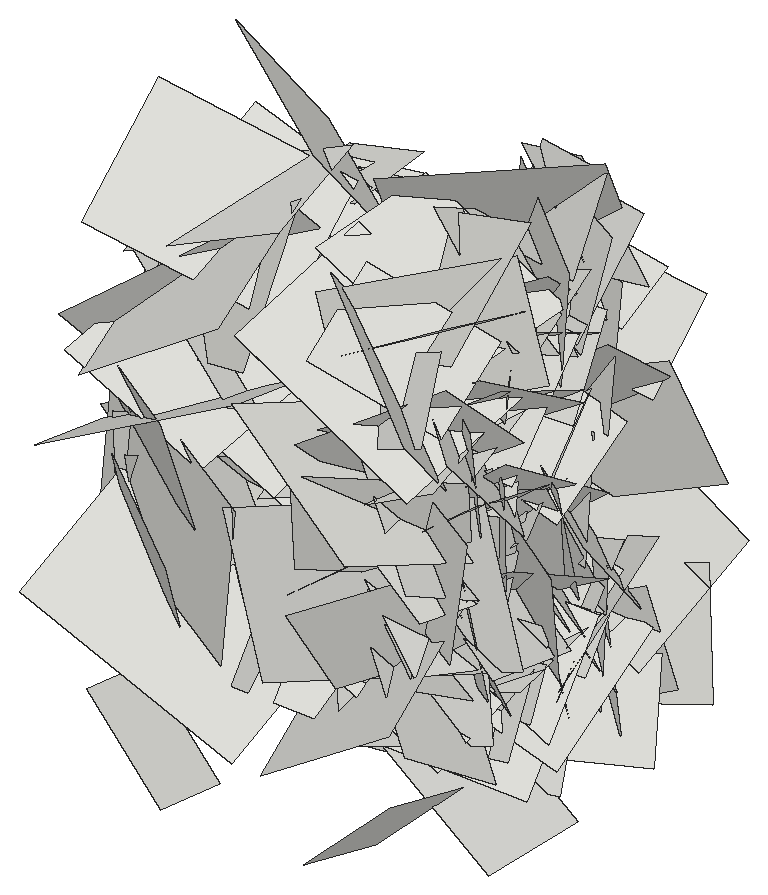
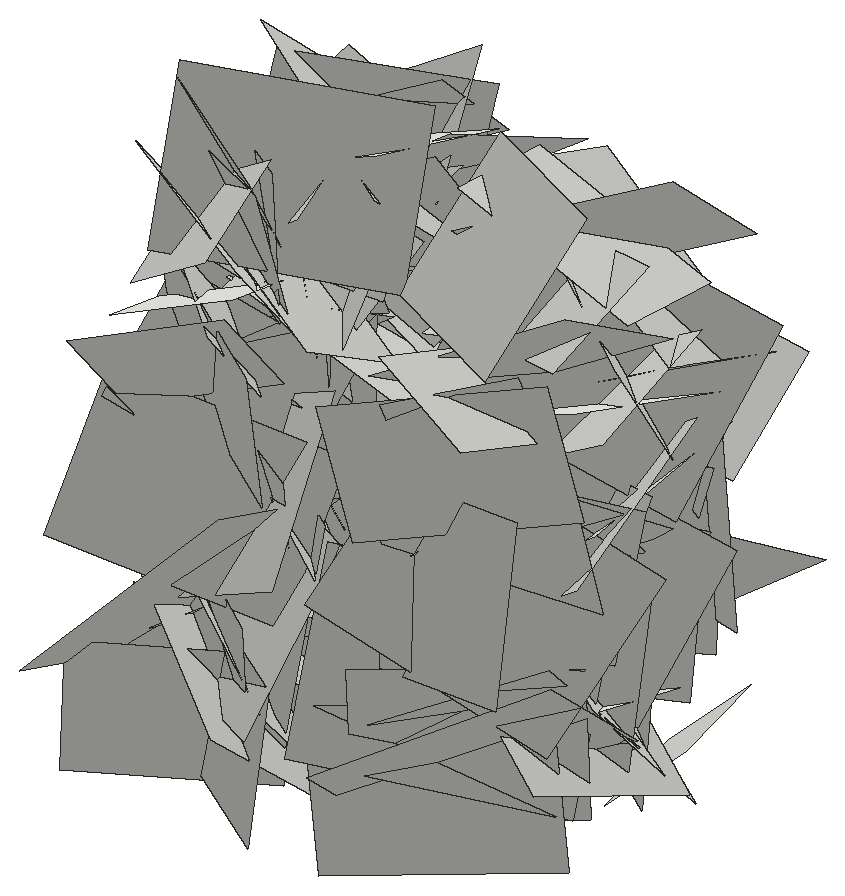
# SketchUp Ruby script. Lengths in inches.
U = 1.inch
M = Sketchup.active_model
def pt(a) = Geom::Point3d.new(a.map { |v| v * U })
def face(e, loops, mat)
  f = e.add_face(loops[0].map { |a| pt(a) })
  loops[1..].each { |l| e.add_face(l.map { |a| pt(a) }).erase! }
  f.material = f.back_material = mat if mat
  f
end
# faces: each face lists its corners as indices into pts; further lists are holes
def faces(e, pts, list, mat = nil) = list.each { |f| face(e, (f[0].is_a?(Array) ? f : [f]).map { |l| l.map { |i| pts[i] } }, mat) }
# xy, xz, yz: faces in a plane at the given z, y or x. An outline is a flat list of corners, or four numbers for a rectangle; further outlines are holes
def ring(l) = l.size == 4 ? [[l[0], l[1]], [l[2], l[1]], [l[2], l[3]], [l[0], l[3]]] : l.each_slice(2).to_a
def flat(e, list, mat, &to3) = list.each { |f| face(e, (f[0].is_a?(Array) ? f : [f]).map { |l| ring(l).map { |u, v| to3.(u, v) } }, mat) }
def xy(e, z, list, mat = nil) = flat(e, list, mat) { |x, y| [x, y, z] }
def xz(e, y, list, mat = nil) = flat(e, list, mat) { |x, z| [x, y, z] }
def yz(e, x, list, mat = nil) = flat(e, list, mat) { |y, z| [x, y, z] }
def lines(e, pts, list) = list.each { |a, b| e.add_line(pt(pts[a]), pt(pts[b])) }
# prism: a flat outline (further loops are holes) pulled along v
def prism(e, loops, v, mat = nil)
  f = face(e, loops, mat); d = Geom::Vector3d.new(v.map { |x| x * U })
  f.pushpull(f.normal.samedirection?(d) ? d.length : -d.length)
end
def box(e, o, s, mat = nil) = prism(e, [[o, [o[0] + s[0], o[1], o[2]], [o[0] + s[0], o[1] + s[1], o[2]], [o[0], o[1] + s[1], o[2]]]], [0, 0, s[2]], mat)
def at(x, y, z, deg = 0) = Geom::Transformation.translation(pt([x, y, z])) * Geom::Transformation.rotation(ORIGIN, Z_AXIS, deg.degrees)
def axes(o, x, y, z) = Geom::Transformation.new([*x, 0, *y, 0, *z, 0, *pt(o).to_a, 1])
def part(name) = M.definitions.add(name)
# library, detail: a bought-in or finely detailed component or shape, given as its bounding box
def library(name, o, s) = part(name).tap { |d| box(d.entities, o, s) }
def detail(e, o, s) = box(e.add_group.entities, o, s)
def put(e, d, t, mat = nil) = e.add_instance(d, t).tap { |i| i.material = mat if mat }
def group(e, t, mat = nil) = e.add_group.tap { |g| g.transformation = t; g.material = mat if mat }.entities
root = M.entities
c1 = part("Component\#6")
p = [[0.01,0,0],[0,3.24,4.54],[4.32,3.24,4.54],[4.33,0,0]]
faces(c1.entities,p,[[0,1,2,3]])
put(root,c1,axes([400.91,193.84,30.46],[0.25587,-1.06575,0.3461],[0.15582,0.3811,1.07099],[1.17751,0.18115,-0.21693]))
put(root,c1,axes([414.68,193.84,30.46],[-0.25587,-1.06575,0.3461],[-0.15582,0.3811,1.07099],[-1.17751,0.18115,-0.21693]))
put(root,c1,axes([404.88,192.39,25.48],[0.15082,-0.34829,0.66058],[0.01541,0.67363,0.35204],[-0.79143,-0.05326,0.13274]))
put(root,c1,axes([410.71,192.39,25.48],[-0.15082,-0.34829,0.66058],[-0.01541,0.67363,0.35204],[0.79143,-0.05326,0.13274]))
put(root,c1,axes([410.71,192.15,39.48],[-0.21361,0.71392,-0.72381],[-0.12034,-0.74908,-0.70723],[1.07091,0.05823,-0.22384]))
put(root,c1,axes([400.91,193.58,33.2],[0.1306,0.22319,-0.86205],[0.05382,-0.87061,-0.21815],[0.94237,0.01879,0.13193]))
put(root,c1,axes([414.68,193.58,33.2],[-0.1306,0.22319,-0.86205],[-0.05382,-0.87061,-0.21815],[-0.94237,0.01879,0.13193]))
put(root,c1,axes([414.68,191.375,35.34],[-0.1473,0.40574,0.51918],[-0.07991,0.51733,-0.42447],[-0.69387,-0.14571,-0.06134]))
put(root,c1,axes([404.88,194.26,19.42],[0.05867,-0.70774,0.13488],[0.12622,0.14241,0.69835],[-0.75321,-0.03127,0.12754]))
put(root,c1,axes([410.71,194.26,19.42],[-0.05867,-0.70774,0.13488],[-0.12622,0.14241,0.69835],[0.75321,-0.03127,0.12754]))
put(root,c1,axes([400.91,194.3,32.47],[-0.23408,0.14056,-1.33491],[0.22407,-1.33233,-0.17526],[1.40507,0.23589,-0.19445]))
put(root,c1,axes([414.68,194.3,32.47],[0.23408,0.14056,-1.33491],[-0.22407,-1.33233,-0.17526],[-1.40507,0.23589,-0.19445]))
put(root,c1,axes([414.68,195.16,37.28],[-0.08536,-0.54597,-0.55526],[-0.06407,-0.55215,0.55168],[-0.82294,0.09962,0.01464]))
put(root,c1,axes([400.91,189.88,26.35],[0.12674,1.17916,0.69894],[-0.07675,0.70605,-1.17877],[1.45096,-0.06565,-0.1234]))
put(root,c1,axes([414.68,189.88,26.35],[-0.12674,1.17916,0.69894],[0.07675,0.70605,-1.17877],[-1.45096,-0.06565,-0.1234]))
put(root,c1,axes([410.71,194.17,31.15],[-0.1572,-0.65225,0.62778],[-0.00257,0.63643,0.66066],[0.9596,-0.10514,0.10461]))
put(root,c1,axes([410.71,192.38,31.46],[0.05244,0.73173,-0.11131],[0.01157,-0.11227,-0.73318],[0.78447,-0.04726,0.01825]))
put(root,c1,axes([400.91,196.54,35.06],[0.17609,-1.11494,-0.45613],[-0.00034,-0.46049,1.12547],[1.27691,0.15363,0.0632]))
put(root,c1,axes([414.68,196.54,35.06],[-0.17609,-1.11494,-0.45613],[0.00034,-0.46049,1.12547],[-1.27691,0.15363,0.0632]))
put(root,c1,axes([414.68,192.76,27.5],[0.21382,-0.08753,1.03604],[-0.20559,1.03367,0.1251],[-1.08277,-0.21355,0.18084]))
put(root,c1,axes([410.71,193.07,33.95],[0.05953,0.85388,-0.40475],[-0.24794,-0.38029,-0.83472],[0.97048,-0.14953,-0.18843]))
put(root,c1,axes([410.71,192.62,23.41],[-0.0945,0.05137,0.75973],[0.00531,0.76494,-0.05113],[0.80713,0.00098,0.08928]))
put(root,c1,axes([400.91,191.97,33.56],[0.08688,0.89449,0.25558],[0.12211,0.24484,-0.89383],[0.97851,-0.10998,0.08885]))
put(root,c1,axes([414.68,191.97,33.56],[-0.08688,0.89449,0.25558],[-0.12211,0.24484,-0.89383],[-0.97851,-0.10998,0.08885]))
put(root,c1,axes([410.71,193.25,29.42],[-0.0602,0.67546,-0.3863],[-0.10598,-0.39045,-0.66802],[0.81797,-0.00088,-0.11498]))
put(root,c1,axes([414.68,194.92,22.54],[-0.07164,-0.895,0.57486],[0.24411,0.55005,0.88344],[-1.1008,0.18023,0.15849]))
put(root,c1,axes([410.71,192.68,25.51],[0.10584,0.56729,0.32604],[-0.07365,0.33715,-0.56532],[0.68964,-0.05105,-0.11041]))
put(root,c1,axes([414.68,195.4,26.27],[-0.15303,-0.80886,0.21466],[0.08059,0.20425,0.82078],[-0.8834,0.15875,0.0377]))
put(root,c1,axes([410.71,192.92,34.17],[-0.15147,-0.1521,1.01718],[-0.1212,1.02293,0.1369],[1.08344,0.09316,0.15752]))
put(root,c1,axes([410.71,195.89,35.57],[-0.03273,-0.74668,0.19464],[0.06894,0.19158,0.74527],[0.81502,-0.04619,-0.05522]))
put(root,c1,axes([410.71,194.0625,27.88],[-0.03826,-0.32146,0.75655],[-0.14724,0.74878,0.31153],[0.85881,0.11405,0.08712]))
put(root,c1,axes([414.68,194.18,31.13],[0.04063,-0.16003,0.87853],[0.02386,0.87924,0.15917],[-0.94627,0.0153,0.04174]))
put(root,c1,axes([400.91,193.85,32.27],[0.12737,1.17977,-0.33684],[-0.1012,-0.32843,-1.18439],[1.29659,-0.14153,-0.05935]))
put(root,c1,axes([414.68,193.85,32.27],[-0.12737,1.17977,-0.33684],[0.1012,-0.32843,-1.18439],[-1.29659,-0.14153,-0.05935]))
put(root,c1,axes([410.71,194.1,30.97],[-0.07757,0.18705,0.69229],[0.05179,0.69557,-0.18277],[0.75837,-0.02837,0.08329]))
put(root,c1,axes([400.91,197.22,25.56],[0.17769,-0.12121,-0.94504],[0.07151,-0.95564,0.13453],[1.00742,0.08922,0.15714]))
put(root,c1,axes([414.68,197.22,25.56],[-0.17769,-0.12121,-0.94504],[-0.07151,-0.95564,0.13453],[-1.00742,0.08922,0.15714]))
put(root,c1,axes([414.68,194.12,36.42],[0.16155,0.92195,-0.51802],[-0.06641,-0.51458,-0.93426],[-1.119,0.16364,-0.01934]))
put(root,c1,axes([414.68,192.77,37.47],[0.01566,0.85002,0.74451],[-0.07038,0.74394,-0.84805],[-1.19569,-0.03266,0.05967]))
put(root,c1,axes([400.91,192.77,37.47],[-0.01566,0.85002,0.74451],[0.07038,0.74394,-0.84805],[1.19569,-0.03266,0.05967]))
put(root,c1,axes([410.71,194.71,36.49],[-0.01491,0.71707,-0.22931],[-0.11795,-0.22881,-0.70868],[0.78925,-0.02064,-0.11024]))
put(root,c1,axes([400.91,198.78,35.93],[0.06513,-0.64723,-0.92238],[0.00055,-0.92374,0.64822],[1.19442,0.03572,0.05]))
put(root,c1,axes([414.68,198.78,35.93],[-0.06513,-0.64723,-0.92238],[-0.00055,-0.92374,0.64822],[-1.19442,0.03572,0.05]))
put(root,c1,axes([400.91,194.52,25.48],[0.11423,-0.20624,1.26777],[0.06819,1.2715,0.20138],[1.3598,-0.04643,-0.1166]))
put(root,c1,axes([414.68,194.52,25.48],[-0.11423,-0.20624,1.26777],[-0.06819,1.2715,0.20138],[-1.3598,-0.04643,-0.1166]))
put(root,c1,axes([400.91,196.22,30.25],[-0.08073,-0.93811,0.99109],[-0.27356,0.98462,0.91216],[1.42044,0.13631,0.232]))
put(root,c1,axes([414.68,196.22,30.25],[0.08073,-0.93811,0.99109],[0.27356,0.98462,0.91216],[-1.42044,0.13631,0.232]))
put(root,c1,axes([400.91,199.72,26.12],[-0.08735,-0.8928,-1.02237],[0.07635,-1.02569,0.88989],[1.43674,0.00023,-0.10945]))
put(root,c1,axes([414.68,199.72,26.12],[0.08735,-0.8928,-1.02237],[-0.07635,-1.02569,0.88989],[-1.43674,0.00023,-0.10945]))
put(root,c1,axes([400.91,193.54,33.12],[0.22081,1.30446,0.31828],[0.37279,0.25784,-1.28691],[1.3736,-0.27967,0.29809]))
put(root,c1,axes([414.68,193.54,33.12],[-0.22081,1.30446,0.31828],[-0.37279,0.25784,-1.28691],[-1.3736,-0.27967,0.29809]))
put(root,c1,axes([400.91,198.24,37.08],[0.15669,-0.99926,-0.19378],[0.22295,-0.1616,0.99377],[1.05566,0.18244,-0.18112]))
put(root,c1,axes([414.68,198.24,37.08],[-0.15669,-0.99926,-0.19378],[-0.22295,-0.1616,0.99377],[-1.05566,0.18244,-0.18112]))
put(root,c1,axes([414.68,197.53,26.62],[-0.11622,-0.11144,-0.6986],[-0.08861,-0.69994,0.12478],[-0.74462,0.10068,0.09418]))
put(root,c1,axes([400.91,195.125,35.61],[0.03117,0.92717,-0.40656],[-0.02653,-0.40594,-0.92757],[1.07281,-0.03698,-0.01113]))
put(root,c1,axes([414.68,195.125,35.61],[-0.03117,0.92717,-0.40656],[0.02653,-0.40594,-0.92757],[-1.07281,-0.03698,-0.01113]))
put(root,c1,axes([400.91,195.34,33.06],[0.01901,1.14103,-0.72029],[-0.19621,-0.71146,-1.13165],[1.41679,-0.11384,-0.14706]))
put(root,c1,axes([414.68,195.34,33.06],[-0.01901,1.14103,-0.72029],[0.19621,-0.71146,-1.13165],[-1.41679,-0.11384,-0.14706]))
put(root,c1,axes([414.68,198.41,25.5],[0.14641,-1.02966,0.26735],[0.10928,0.28128,1.03005],[-1.12233,-0.10694,0.13517]))
put(root,c1,axes([414.68,198.72,19.65],[0.06387,-1.04135,0.05905],[0.06023,0.06234,1.04135],[-1.10396,-0.05685,0.06023]))
put(root,c1,axes([400.91,195.625,24.52],[0.22176,-0.47224,1.18941],[0.10161,1.2076,0.46259],[1.3527,-0.0133,-0.22974]))
put(root,c1,axes([414.68,195.625,24.52],[-0.22176,-0.47224,1.18941],[-0.10161,1.2076,0.46259],[-1.3527,-0.0133,-0.22974]))
put(root,c1,axes([404.88,196.3,29.33],[0.09147,0.43894,-0.4809],[-0.05464,-0.47898,-0.44644],[-0.688,0.09639,-0.02848]))
put(root,c1,axes([410.71,196.3,29.33],[-0.09147,0.43894,-0.4809],[0.05464,-0.47898,-0.44644],[0.688,0.09639,-0.02848]))
put(root,c1,axes([414.68,195.45,23.05],[-0.08121,0.42866,0.62692],[-0.16296,0.6083,-0.43472],[-0.78836,-0.1699,0.02528]))
put(root,c1,axes([400.91,195.04,27.27],[0.2131,0.57774,0.71728],[0.02179,0.73117,-0.59469],[0.97604,-0.14247,-0.14333]))
put(root,c1,axes([414.68,195.04,27.27],[-0.2131,0.57774,0.71728],[-0.02179,0.73117,-0.59469],[-0.97604,-0.14247,-0.14333]))
put(root,c1,axes([410.71,198.57,33.25],[-0.09717,0.14422,-0.89801],[-0.11089,-0.89824,-0.13357],[0.95769,-0.08937,-0.10658]))
put(root,c1,axes([400.91,197.21,31.46],[0.04455,0.58157,-0.95839],[0.2239,-0.94599,-0.56478],[1.16701,0.1593,0.14494]))
put(root,c1,axes([414.68,197.21,31.46],[-0.04455,0.58157,-0.95839],[-0.2239,-0.94599,-0.56478],[-1.16701,0.1593,0.14494]))
put(root,c1,axes([414.68,195.7,29.31],[0.12944,0.87645,-0.3909],[-0.13192,-0.37627,-0.88251],[-1.00866,0.16168,0.06525]))
put(root,c1,axes([400.91,197.34,38.49],[0.22162,0.66132,-0.53694],[-0.02723,-0.54773,-0.68462],[0.90256,-0.17891,0.1112]))
put(root,c1,axes([414.68,197.34,38.49],[-0.22162,0.66132,-0.53694],[0.02723,-0.54773,-0.68462],[-0.90256,-0.17891,0.1112]))
put(root,c1,axes([414.68,196.41,37.05],[-0.02372,0.78814,-0.36288],[-0.15491,-0.36124,-0.77556],[-0.90659,0.0411,0.14202]))
put(root,c1,axes([414.68,195.33,34.42],[-0.12228,0.30682,0.85432],[0.19875,0.85067,-0.2802],[-0.94146,0.13973,-0.17012]))
put(root,c1,axes([414.68,200.17,25.9],[-0.12286,-0.34825,-0.84521],[0.12526,-0.85054,0.33424],[-0.96086,-0.06635,0.15165]))
put(root,c1,axes([414.68,197.85,24.73],[0.35143,-0.52734,1.13432],[-0.18025,1.14359,0.58135],[-1.31365,-0.29799,0.22369]))
put(root,c1,axes([400.91,197.85,24.73],[-0.35143,-0.52734,1.13432],[0.18025,1.14359,0.58135],[1.31365,-0.29799,0.22369]))
put(root,c1,axes([410.71,196.95,39.61],[-0.06663,0.78722,-0.39485],[-0.0883,-0.3994,-0.78302],[0.92935,0.01849,-0.10271]))
put(root,c1,axes([400.91,202.23,24.6],[-0.19755,-1.2824,-0.48224],[-0.04087,-0.48158,1.29554],[1.4517,-0.18807,-0.02915]))
put(root,c1,axes([414.68,202.23,24.6],[0.19755,-1.2824,-0.48224],[0.04087,-0.48158,1.29554],[-1.4517,-0.18807,-0.02915]))
put(root,c1,axes([410.71,199.74,34.07],[0.11183,-0.60219,-0.2199],[-0.02555,-0.22643,0.6085],[0.67907,0.09065,0.0591]))
put(root,c1,axes([410.71,197.11,20.7],[-0.0234,0.20043,0.60552],[0.11848,0.59772,-0.19378],[0.66563,-0.09934,0.05578]))
put(root,c1,axes([414.68,201.02,32],[0.03236,-0.79816,-0.43551],[0.07074,-0.43262,0.79753],[-0.9612,-0.0587,0.04403]))
put(root,c1,axes([414.68,200.08,36.17],[-0.04967,-0.3024,-0.77978],[-0.15753,-0.76557,0.30582],[-0.87244,0.15545,-0.01082]))
put(root,c1,axes([400.91,196.04,25.17],[0.02819,1.07686,0.22249],[0.25409,0.21152,-1.05244],[1.13755,-0.07393,0.22957]))
put(root,c1,axes([414.68,196.04,25.17],[-0.02819,1.07686,0.22249],[-0.25409,0.21152,-1.05244],[-1.13755,-0.07393,0.22957]))
put(root,c1,axes([400.91,196.35,35.86],[0.06555,0.97369,0.5362],[0.0688,0.53295,-0.97527],[1.17625,-0.08544,0.02716]))
put(root,c1,axes([414.68,196.35,35.86],[-0.06555,0.97369,0.5362],[-0.0688,0.53295,-0.97527],[-1.17625,-0.08544,0.02716]))
put(root,c1,axes([410.71,196.5,26.6],[-0.00001,0.64808,0.59207],[-0.20568,0.57742,-0.63205],[0.90746,0.13088,-0.14325]))
put(root,c1,axes([400.91,196.35,30.1],[0.25467,1.00338,0.64071],[-0.12934,0.67094,-1.00496],[1.25528,-0.13443,-0.23354]))
put(root,c1,axes([414.68,196.35,30.1],[-0.25467,1.00338,0.64071],[0.12934,0.67094,-1.00496],[-1.25528,-0.13443,-0.23354]))
put(root,c1,axes([410.71,198.68,37.125],[0.06347,0.58127,-0.24952],[-0.07215,-0.24326,-0.58302],[0.66662,-0.08167,-0.03935]))
put(root,c1,axes([410.71,201.02,39.48],[-0.13577,0.09163,-0.9618],[-0.05798,-0.96935,-0.08506],[1.02248,-0.0428,-0.13253]))
put(root,c1,axes([414.68,199.18,25.47],[-0.11604,-0.3767,0.6399],[0.02749,0.64448,0.38383],[-0.78661,0.07809,-0.08099]))
put(root,c1,axes([400.91,199.97,41.09],[0.2759,0.65189,-0.94787],[0.07756,-0.97924,-0.65337],[1.21695,-0.08538,0.25653]))
put(root,c1,axes([414.68,199.97,41.09],[-0.2759,0.65189,-0.94787],[-0.07756,-0.97924,-0.65337],[-1.21695,-0.08538,0.25653]))
put(root,c1,axes([400.91,198.8,27.02],[-0.0226,-0.2767,0.96977],[0.06915,0.96758,0.27751],[1.06674,-0.06859,0.00256]))
put(root,c1,axes([414.68,198.8,27.02],[0.0226,-0.2767,0.96977],[-0.06915,0.96758,0.27751],[-1.06674,-0.06859,0.00256]))
put(root,c1,axes([400.91,198.29,23.22],[0.04433,-0.32511,1.32538],[-0.126,1.3201,0.32757],[1.44106,0.12543,-0.01213]))
put(root,c1,axes([414.68,198.29,23.22],[-0.04433,-0.32511,1.32538],[0.126,1.3201,0.32757],[-1.44106,0.12543,-0.01213]))
put(root,c1,axes([410.71,197.17,21.41],[-0.31691,0.51794,0.91951],[-0.05422,0.94746,-0.55031],[1.11735,0.19287,0.23409]))
put(root,c1,axes([410.71,202.06,39.63],[-0.00244,-0.36914,-0.6705],[0.07457,-0.66776,0.36739],[0.80789,0.06052,-0.03594]))
put(root,c1,axes([414.68,198.86,35.2],[0.14047,0.16017,0.87964],[-0.13868,0.88315,-0.1411],[-0.93754,-0.10664,0.15267]))
put(root,c1,axes([414.68,200.1,34.99],[-0.01875,0.74709,-0.59948],[0.09315,-0.59579,-0.74508],[-1.01106,-0.06874,-0.05753]))
put(root,c1,axes([400.91,199.05,27.98],[0.08019,0.19915,0.92966],[0.13728,0.92174,-0.20799],[0.9984,-0.14274,-0.04607]))
put(root,c1,axes([414.68,199.05,27.98],[-0.08019,0.19915,0.92966],[-0.13728,0.92174,-0.20799],[-0.9984,-0.14274,-0.04607]))
put(root,c1,axes([400.91,197.73,24.08],[0.06299,0.80841,0.87356],[-0.01823,0.87514,-0.8087],[1.26151,-0.02772,-0.0553]))
put(root,c1,axes([414.68,197.73,24.08],[-0.06299,0.80841,0.87356],[0.01823,0.87514,-0.8087],[-1.26151,-0.02772,-0.0553]))
put(root,c1,axes([414.68,201.91,26.14],[0.02369,0.31708,-0.9382],[0.09459,-0.93526,-0.31396],[-1.04548,-0.07743,-0.04967]))
put(root,c1,axes([400.91,201.66,25.46],[-0.21728,-0.88431,0.94199],[0.03627,0.94972,0.89901],[1.36907,-0.16551,0.12568]))
put(root,c1,axes([414.68,201.66,25.46],[0.21728,-0.88431,0.94199],[-0.03627,0.94972,0.89901],[-1.36907,-0.16551,0.12568]))
put(root,c1,axes([414.68,198.67,35.61],[0.10111,0.59855,0.78971],[-0.15679,0.79307,-0.58323],[-1.03859,-0.06146,0.16492]))
put(root,c1,axes([400.91,200.57,23.13],[0.2198,-0.69796,1.13548],[-0.0671,1.14269,0.71395],[1.41122,0.16304,-0.1429]))
put(root,c1,axes([414.68,200.57,23.13],[-0.2198,-0.69796,1.13548],[0.0671,1.14269,0.71395],[-1.41122,0.16304,-0.1429]))
put(root,c1,axes([400.91,197.83,24.35],[-0.09568,0.96283,0.81475],[-0.1112,0.80827,-0.9668],[1.33234,0.1366,-0.02218]))
put(root,c1,axes([414.68,197.83,24.35],[0.09568,0.96283,0.81475],[0.1112,0.80827,-0.9668],[-1.33234,0.1366,-0.02218]))
put(root,c1,axes([400.91,199.8,22.82],[-0.00598,0.07204,1.08492],[-0.02761,1.08461,-0.07215],[1.15221,0.02636,0.0039]))
put(root,c1,axes([414.68,199.8,22.82],[0.00598,0.07204,1.08492],[0.02761,1.08461,-0.07215],[-1.15221,0.02636,0.0039]))
put(root,c1,axes([410.71,201.07,39.9375],[-0.03161,0.68058,-0.41337],[-0.06223,-0.41441,-0.67806],[0.84176,-0.00508,-0.06565]))
put(root,c1,axes([404.88,203.75,35.72],[0.12855,-0.35471,-0.52952],[0.05195,-0.53223,0.36775],[-0.67359,-0.10874,-0.07269]))
put(root,c1,axes([410.71,203.75,35.72],[-0.12855,-0.35471,-0.52952],[-0.05195,-0.53223,0.36775],[0.67359,-0.10874,-0.07269]))
put(root,c1,axes([400.91,200.11,31.93],[0.08158,0.26048,1.04137],[0.05734,1.04178,-0.26458],[1.13642,-0.07126,-0.06141]))
put(root,c1,axes([414.68,200.11,31.93],[-0.08158,0.26048,1.04137],[-0.05734,1.04178,-0.26458],[-1.13642,-0.07126,-0.06141]))
put(root,c1,axes([404.88,200.57,36.04],[0.10099,0.61602,0.17436],[-0.1325,0.19079,-0.60575],[-0.66557,0.05549,0.14705]))
put(root,c1,axes([410.71,200.57,36.04],[-0.10099,0.61602,0.17436],[0.1325,0.19079,-0.60575],[0.66557,0.05549,0.14705]))
put(root,c1,axes([400.91,200.75,21.625],[0.14431,-0.01788,1.13958],[0.06693,1.14604,0.01044],[1.20625,-0.06145,-0.13692]))
put(root,c1,axes([414.68,200.75,21.625],[-0.14431,-0.01788,1.13958],[-0.06693,1.14604,0.01044],[-1.20625,-0.06145,-0.13692]))
put(root,c1,axes([400.91,202.95,33.21],[-0.17447,0.42234,-1.07867],[0.17991,-1.06896,-0.44444],[1.21466,0.21899,-0.08911]))
put(root,c1,axes([414.68,202.95,33.21],[0.17447,0.42234,-1.07867],[-0.17991,-1.06896,-0.44444],[-1.21466,0.21899,-0.08911]))
put(root,c1,axes([414.68,206.72,25.52],[0.07134,-1.27871,-0.42932],[0.37284,-0.39835,1.24159],[-1.38032,-0.17369,0.31318]))
put(root,c1,axes([414.68,204.82,25.65],[0.12938,-0.11687,-1.00907],[-0.02351,-1.01639,0.11504],[-1.07651,0.00815,-0.12379]))
put(root,c1,axes([414.68,204.74,34.65],[-0.08046,-0.48471,-0.63269],[-0.12911,-0.62103,0.49039],[-0.83492,0.14274,-0.01486]))
